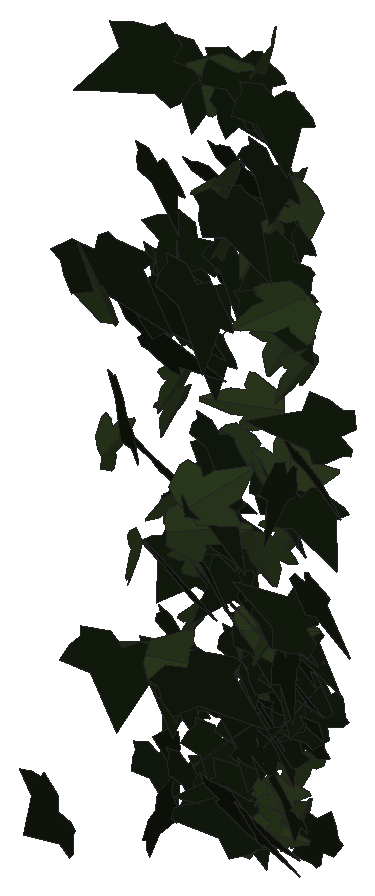
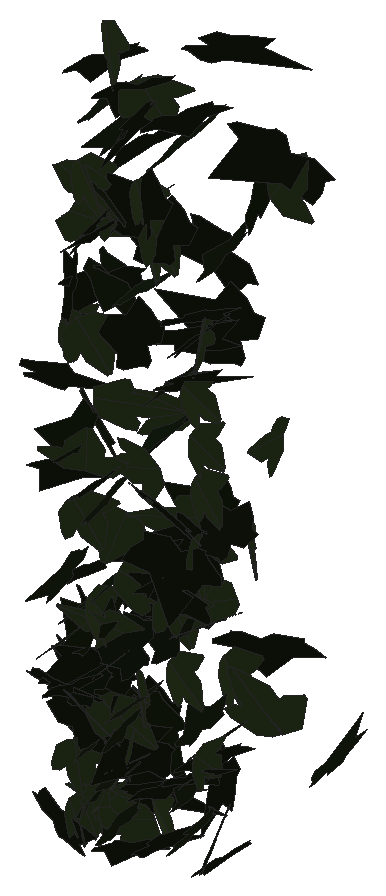
# SketchUp Ruby script. Lengths in inches.
U = 1.inch
M = Sketchup.active_model
def pt(a) = Geom::Point3d.new(a.map { |v| v * U })
def face(e, loops, mat)
  f = e.add_face(loops[0].map { |a| pt(a) })
  loops[1..].each { |l| e.add_face(l.map { |a| pt(a) }).erase! }
  f.material = f.back_material = mat if mat
  f
end
# faces: each face lists its corners as indices into pts; further lists are holes
def faces(e, pts, list, mat = nil) = list.each { |f| face(e, (f[0].is_a?(Array) ? f : [f]).map { |l| l.map { |i| pts[i] } }, mat) }
# xy, xz, yz: faces in a plane at the given z, y or x. An outline is a flat list of corners, or four numbers for a rectangle; further outlines are holes
def ring(l) = l.size == 4 ? [[l[0], l[1]], [l[2], l[1]], [l[2], l[3]], [l[0], l[3]]] : l.each_slice(2).to_a
def flat(e, list, mat, &to3) = list.each { |f| face(e, (f[0].is_a?(Array) ? f : [f]).map { |l| ring(l).map { |u, v| to3.(u, v) } }, mat) }
def xy(e, z, list, mat = nil) = flat(e, list, mat) { |x, y| [x, y, z] }
def xz(e, y, list, mat = nil) = flat(e, list, mat) { |x, z| [x, y, z] }
def yz(e, x, list, mat = nil) = flat(e, list, mat) { |y, z| [x, y, z] }
def lines(e, pts, list) = list.each { |a, b| e.add_line(pt(pts[a]), pt(pts[b])) }
# prism: a flat outline (further loops are holes) pulled along v
def prism(e, loops, v, mat = nil)
  f = face(e, loops, mat); d = Geom::Vector3d.new(v.map { |x| x * U })
  f.pushpull(f.normal.samedirection?(d) ? d.length : -d.length)
end
def box(e, o, s, mat = nil) = prism(e, [[o, [o[0] + s[0], o[1], o[2]], [o[0] + s[0], o[1] + s[1], o[2]], [o[0], o[1] + s[1], o[2]]]], [0, 0, s[2]], mat)
def at(x, y, z, deg = 0) = Geom::Transformation.translation(pt([x, y, z])) * Geom::Transformation.rotation(ORIGIN, Z_AXIS, deg.degrees)
def axes(o, x, y, z) = Geom::Transformation.new([*x, 0, *y, 0, *z, 0, *pt(o).to_a, 1])
def part(name) = M.definitions.add(name)
# library, detail: a bought-in or finely detailed component or shape, given as its bounding box
def library(name, o, s) = part(name).tap { |d| box(d.entities, o, s) }
def detail(e, o, s) = box(e.add_group.entities, o, s)
def put(e, d, t, mat = nil) = e.add_instance(d, t).tap { |i| i.material = mat if mat }
def group(e, t, mat = nil) = e.add_group.tap { |g| g.transformation = t; g.material = mat if mat }.entities
root = M.entities
M.materials.add("1026 AP 7946 SUNNY SIDE UP").color = [254, 231, 186]
M.materials.add("efeu1").color = [18, 25, 13]
M.materials.add("efeu2").color = [43, 57, 29]
c1 = part("ivyleaf_10")
p = [[0,0.5,-0.03],[-0.0625,2.02,-0.43],[-0.19,2.01,-0.46],[-0.54,1.05,-0.29],[-0.52,0.625,-0.18],[-0.83,0.76,-0.28],
  [-1.16,0.64,-0.33],[-1.15,0.33,-0.24],[-0.77,-0.39,0.02],[-0.3,-0.51,0.16],[0.04,-0.48,0.23],[-0.02,2.01,-0.4375],
  [-0.06,2.01,-0.43],[0.04,-0.49,0.23],[0.67,-0.49,0.14],[1.38,0.36,-0.2],[1.375,0.51,-0.24],[0.81,0.65,-0.19],
  [0.62,0.59,-0.15],[0.6,1.09,-0.28],[0.5,1.23,-0.31]]
faces(c1.entities,p,[[0,1,2,3,4,5,6,7,8,9,10],[11,12,0,13,14,15,16,17,18,19,20]],"efeu2")
c2 = part("ivyleaf_9")
p = [[1.54,2.16,1.25],[1.36,2.04,1.19],[-0.21,0.99,0.68],[-0.71,1.11,0.82],[-0.85,0.86,0.67],[-0.8,0.17,0.21],
  [-0.9,-0.01,0.1],[-0.67,-0.16,-0.02],[-0.08,-0.08,-0.05],[-0.03,-0.6,-0.4],[0.65,-0.88,-0.66],[0.83,-0.6,-0.49],
  [1.29,-0.42,-0.43],[1.8125,-0.07,-0.26],[1.21,0.44,0.15]]
faces(c2.entities,p,[[0,1,2,3,4,5,6,7,8,9,10,11,12,13,14]],"efeu1")
put(root,c1,axes([108.21,211.42,269.92],[-0.38508,-0.11974,0.18421],[0.25693,0.07439,0.28124],[-0.22157,0.29438,0.00598]),"1026 AP 7946 SUNNY SIDE UP")
put(root,c2,axes([108.45,212.45,268.24],[-0.09112,0.03942,0.27025],[-0.12592,-0.25836,0.02028],[0.39729,-0.07284,0.06841]),"1026 AP 7946 SUNNY SIDE UP")
put(root,c2,axes([108.26,212.3125,276.96],[0.1139,-0.28352,0.10218],[0.01275,-0.1018,-0.30159],[0.47298,0.07102,-0.01647]),"1026 AP 7946 SUNNY SIDE UP")
put(root,c1,axes([108.5,212.45,273.58],[0.01567,-0.27591,0.10372],[0.02815,-0.10155,-0.28469],[0.46182,0.01555,0.01384]),"1026 AP 7946 SUNNY SIDE UP")
put(root,c2,axes([108.35,212.22,268.26],[0.03152,-0.26953,-0.01684],[0,0.01486,-0.27835],[0.42445,0.02002,0.00125]),"1026 AP 7946 SUNNY SIDE UP")
put(root,c1,axes([108.45,212.51,269.73],[-0.0271,-0.18167,0.22393],[0.11944,-0.21378,-0.17827],[0.43042,0.04789,0.06357]),"1026 AP 7946 SUNNY SIDE UP")
put(root,c2,axes([108.48,209.94,268.49],[-0.15512,-0.1523,0.33154],[-0.07342,-0.3264,-0.17532],[0.55625,-0.08556,0.06931]),"1026 AP 7946 SUNNY SIDE UP")
put(root,c1,axes([108.59,210.81,273.55],[0.01808,0.03987,-0.32698],[0.09158,0.31227,0.04438],[0.49495,-0.05923,0.00374]),"1026 AP 7946 SUNNY SIDE UP")
put(root,c1,axes([108.64,212.47,274.91],[0.03982,-0.23204,0.18636],[0.02591,-0.18149,-0.24152],[0.4632,0.0301,-0.00251]),"1026 AP 7946 SUNNY SIDE UP")
put(root,c2,axes([108.54,212.25,269.64],[-0.10608,-0.28832,-0.00645],[0.01244,0.0029,-0.30494],[0.45324,-0.06756,0.00686]),"1026 AP 7946 SUNNY SIDE UP")
put(root,c2,axes([108.5,212.14,269.85],[0.02076,-0.27844,0.0287],[-0.00017,-0.02948,-0.28733],[0.44026,0.01312,-0.00146]),"1026 AP 7946 SUNNY SIDE UP")
put(root,c2,axes([108.36,212.08,272.72],[0.02547,-0.15199,0.26034],[0.2298,-0.21663,-0.14466],[0.40408,0.13278,0.06586]),"1026 AP 7946 SUNNY SIDE UP")
put(root,c1,axes([108.64,212.22,275.74],[0.10842,-0.25066,-0.15622],[0.06657,0.16128,-0.25628],[0.45464,0.03616,0.07478]),"1026 AP 7946 SUNNY SIDE UP")
put(root,c2,axes([108.85,212.52,275.01],[-0.31926,-0.0955,0.20724],[-0.20456,-0.17092,-0.21927],[0.28513,-0.22956,0.07473]),"1026 AP 7946 SUNNY SIDE UP")
put(root,c1,axes([108.6875,212.27,274.09],[0.00841,-0.22697,0.19007],[0.05005,-0.18427,-0.23394],[0.45848,0.02428,0.02205]),"1026 AP 7946 SUNNY SIDE UP")
put(root,c2,axes([108.74,212.47,275.97],[-0.29125,-0.2036,0.1153],[-0.04572,-0.12313,-0.27819],[0.36333,-0.1787,0.05742]),"1026 AP 7946 SUNNY SIDE UP")
put(root,c2,axes([108.72,212.46,269.38],[-0.22926,-0.20854,0.0696],[-0.01866,-0.07491,-0.26049],[0.34476,-0.14273,0.03218]),"1026 AP 7946 SUNNY SIDE UP")
put(root,c2,axes([108.56,212.39,270.1],[0.02886,-0.22884,0.17961],[0.06645,-0.17196,-0.23637],[0.44871,0.04019,0.02346]),"1026 AP 7946 SUNNY SIDE UP")
put(root,c2,axes([108.59,212.24,269.48],[0.11709,-0.26504,-0.00957],[-0.0023,0.00768,-0.28356],[0.41692,0.07448,0.00112]),"1026 AP 7946 SUNNY SIDE UP")
put(root,c2,axes([108.625,212.42,269.23],[0.11304,-0.25356,0.08159],[0.01761,-0.08057,-0.27176],[0.41801,0.07197,-0.01061]),"1026 AP 7946 SUNNY SIDE UP")
put(root,c2,axes([108.8,212.22,271.37],[-0.20416,-0.21499,0.13414],[-0.01633,-0.14316,-0.25266],[0.39588,-0.11678,0.05875]),"1026 AP 7946 SUNNY SIDE UP")
put(root,c1,axes([108.85,211.95,272.4],[-0.08755,-0.29398,-0.07375],[0.04188,0.06604,-0.30754],[0.47331,-0.06022,0.01357]),"1026 AP 7946 SUNNY SIDE UP")
put(root,c2,axes([108.67,212.25,275.67],[0.08604,-0.298,-0.03228],[-0.0153,0.02834,-0.31193],[0.47064,0.0554,-0.00424]),"1026 AP 7946 SUNNY SIDE UP")
put(root,c2,axes([109.18,211.39,279.24],[-0.46035,-0.12319,0.18772],[-0.24253,-0.10291,-0.32633],[0.24784,-0.32952,0.02935]),"1026 AP 7946 SUNNY SIDE UP")
put(root,c2,axes([108.83,210.85,270.6],[-0.32112,-0.25471,-0.11661],[0.1453,0.06862,-0.33472],[0.41251,-0.22245,0.02713]),"1026 AP 7946 SUNNY SIDE UP")
put(root,c1,axes([108.98,211.25,270.29],[0.02619,-0.33234,0.09783],[0.0047,-0.09682,-0.34337],[0.5443,0.01683,-0.00174]),"1026 AP 7946 SUNNY SIDE UP")
put(root,c2,axes([109.28,211.97,275.2],[-0.4254,-0.19819,0.01138],[-0.00316,0.02331,0.34502],[-0.31221,0.26981,-0.01901]),"1026 AP 7946 SUNNY SIDE UP")
put(root,c1,axes([109.04,212.26,270.68],[0.03283,-0.26956,0.13359],[0.01045,-0.13107,-0.27928],[0.47129,0.02168,-0.00311]),"1026 AP 7946 SUNNY SIDE UP")
put(root,c2,axes([109.02,212.26,272.37],[0.32245,0.19273,-0.10985],[-0.09658,-0.09142,-0.28949],[-0.33347,0.21284,-0.02238]),"1026 AP 7946 SUNNY SIDE UP")
put(root,c1,axes([109.0625,210.85,272.1875],[0.2021,-0.2708,-0.1119],[-0.0382,0.10667,-0.30732],[0.45629,0.12887,0.02383]),"1026 AP 7946 SUNNY SIDE UP")
put(root,c2,axes([108.9375,212.37,278.75],[-0.17368,-0.30751,0.00823],[0.00534,-0.01156,-0.3366],[0.48375,-0.11028,0.00667]),"1026 AP 7946 SUNNY SIDE UP")
put(root,c1,axes([109.14,212.23,271.58],[-0.18566,-0.24349,0.08926],[-0.02236,-0.09051,-0.27808],[0.4065,-0.11618,0.02547]),"1026 AP 7946 SUNNY SIDE UP")
put(root,c2,axes([108.92,212.11,268.35],[0.09409,-0.25828,0.0604],[0.00915,-0.06031,-0.27336],[0.41687,0.05962,-0.00763]),"1026 AP 7946 SUNNY SIDE UP")
put(root,c1,axes([109.41,209.74,276.38],[-0.41079,0.20274,-0.18884],[-0.19518,0.13968,0.3401],[0.38426,0.28769,-0.02913]),"1026 AP 7946 SUNNY SIDE UP")
put(root,c1,axes([109.26,212.43,276.96],[-0.07602,-0.27745,0.10971],[0.00885,-0.11031,-0.28983],[0.46811,-0.04297,0.0233]),"1026 AP 7946 SUNNY SIDE UP")
put(root,c2,axes([109.05,212.37,271.9],[-0.22818,-0.12076,-0.23174],[0.31956,0.10069,-0.19074],[0.24142,-0.24741,0.03345]),"1026 AP 7946 SUNNY SIDE UP")
put(root,c2,axes([108.89,211.95,272.35],[0.0601,-0.04519,-0.31088],[0.47289,0.05549,0.03104],[0.07873,-0.29882,0.05093]),"1026 AP 7946 SUNNY SIDE UP")
put(root,c2,axes([109.35,212.39,268.15],[-0.2095,-0.1547,0.18511],[-0.14566,-0.15686,-0.20978],[0.34434,-0.16047,0.02389]),"1026 AP 7946 SUNNY SIDE UP")
put(root,c2,axes([109.14,212.22,271.95],[-0.04668,-0.26512,-0.10814],[0.03026,0.10192,-0.27413],[0.44647,-0.03463,0.00728]),"1026 AP 7946 SUNNY SIDE UP")
put(root,c2,axes([109.49,212.27,273.01],[-0.47,0.07295,-0.05335],[0.06885,-0.03984,-0.31589],[-0.12311,-0.3008,0.02701]),"1026 AP 7946 SUNNY SIDE UP")
put(root,c2,axes([109.14,212.25,274.76],[0.01013,-0.28119,0.09487],[0.01244,-0.09351,-0.29025],[0.46588,0.00861,0.00569]),"1026 AP 7946 SUNNY SIDE UP")
put(root,c2,axes([108.88,211.29,275.11],[0.24269,-0.12626,0.30548],[0.33277,-0.20931,-0.20603],[0.38358,0.26147,-0.01454]),"1026 AP 7946 SUNNY SIDE UP")
put(root,c2,axes([109.06,212.26,271.18],[0.2126,-0.22558,0.15947],[0.10003,-0.14348,-0.27124],[0.41957,0.14851,-0.01614]),"1026 AP 7946 SUNNY SIDE UP")
put(root,c1,axes([109.73,212.28,271.75],[-0.15956,0.00118,0.30737],[-0.43561,-0.11735,-0.09728],[0.17414,-0.29247,0.03828]),"1026 AP 7946 SUNNY SIDE UP")
put(root,c2,axes([109.5,210.74,268.5],[0.0177,-0.00007,-0.35622],[-0.37138,0.25267,-0.0065],[0.39709,0.23632,0.0098]),"1026 AP 7946 SUNNY SIDE UP")
put(root,c2,axes([109.04,212.43,276.92],[0.17425,-0.14442,0.25797],[0.30636,-0.16197,-0.1854],[0.33729,0.22173,0.03513]),"1026 AP 7946 SUNNY SIDE UP")
put(root,c1,axes([109.56,212.26,278.84],[-0.30468,-0.20546,0.14914],[-0.02088,-0.1755,-0.27374],[0.39572,-0.16745,0.10038]),"1026 AP 7946 SUNNY SIDE UP")
put(root,c2,axes([109.26,212.06,271.52],[0.06623,-0.20026,0.20276],[0.08537,-0.19063,-0.21168],[0.43446,0.06798,0.01069]),"1026 AP 7946 SUNNY SIDE UP")
put(root,c2,axes([109.41,212.1875,268.88],[-0.1118,-0.26349,0.02848],[-0.00094,-0.03001,-0.28123],[0.41683,-0.07074,0.00701]),"1026 AP 7946 SUNNY SIDE UP")
put(root,c1,axes([109.55,212.35,277.39],[0.01457,-0.31132,0.0107],[-0.00388,-0.01224,-0.32092],[0.48987,0.00916,-0.00286]),"1026 AP 7946 SUNNY SIDE UP")
put(root,c2,axes([109.18,209.91,277.04],[-0.11236,-0.0908,-0.37005],[0.43755,0.22759,-0.11513],[0.38345,-0.2863,0.02293]),"1026 AP 7946 SUNNY SIDE UP")
put(root,c1,axes([109.65,211.87,268.35],[0.14164,-0.26064,0.03875],[0.00591,-0.04004,-0.28417],[0.41438,0.08966,-0.00919]),"1026 AP 7946 SUNNY SIDE UP")
put(root,c1,axes([109.71,212,276.66],[0.07654,-0.29666,-0.08718],[-0.0175,0.08222,-0.30921],[0.48403,0.04988,0.0026]),"1026 AP 7946 SUNNY SIDE UP")
put(root,c2,axes([109.55,212.22,278.56],[0.19127,-0.19571,-0.25033],[-0.17569,0.21491,-0.23576],[0.45661,0.16468,0.01415]),"1026 AP 7946 SUNNY SIDE UP")
put(root,c1,axes([109.6875,212.21,270.34],[0.21161,-0.22872,-0.09366],[-0.00651,0.10006,-0.2689],[0.38621,0.12701,0.04678]),"1026 AP 7946 SUNNY SIDE UP")
put(root,c2,axes([109.54,212.54,270.16],[0.00895,-0.26353,0.08883],[0.0243,-0.0873,-0.27174],[0.43605,0.01027,0.01332]),"1026 AP 7946 SUNNY SIDE UP")
put(root,c1,axes([109.4,211.4,272.37],[0.03938,-0.01328,-0.34519],[0.42802,0.19691,0.01407],[0.30774,-0.27217,0.02459]),"1026 AP 7946 SUNNY SIDE UP")
put(root,c2,axes([109.32,210.91,276.02],[0.05322,-0.068,-0.32864],[0.47655,0.12411,0.00661],[0.18797,-0.2954,0.0763]),"1026 AP 7946 SUNNY SIDE UP")
put(root,c2,axes([109.6,212.34,275.97],[-0.07769,-0.26625,0.12791],[0.03977,-0.13079,-0.27599],[0.46123,-0.03357,0.04534]),"1026 AP 7946 SUNNY SIDE UP")
put(root,c2,axes([109.37,212.47,277.19],[0.14324,-0.11433,0.28617],[0.26654,-0.2209,-0.15187],[0.39109,0.19242,-0.00131]),"1026 AP 7946 SUNNY SIDE UP")
put(root,c2,axes([109.58,212.21,269.48],[0.36551,0.14994,0.05592],[0.08399,0.0156,-0.28443],[-0.23577,0.238,-0.01463]),"1026 AP 7946 SUNNY SIDE UP")
put(root,c2,axes([109.58,212.0625,272.18],[0.00854,-0.25532,-0.13761],[0.0296,0.13218,-0.26157],[0.45107,-0.00384,0.01977]),"1026 AP 7946 SUNNY SIDE UP")
put(root,c2,axes([109.62,212.36,278.94],[-0.09019,-0.28228,-0.11128],[0.05527,0.10133,-0.29583],[0.47112,-0.06593,0.0134]),"1026 AP 7946 SUNNY SIDE UP")
put(root,c2,axes([109.42,212.47,275.35],[0.24084,-0.14711,0.22529],[0.2246,-0.16738,-0.21921],[0.34959,0.20889,-0.01438]),"1026 AP 7946 SUNNY SIDE UP")
put(root,c1,axes([110.06,212.36,269.84],[-0.25809,-0.08493,0.22107],[-0.27365,-0.1283,-0.18977],[0.23942,-0.23819,0.02141]),"1026 AP 7946 SUNNY SIDE UP")
put(root,c2,axes([109.66,211.84,273.63],[0.00195,-0.26567,0.12454],[0.03045,-0.12206,-0.27385],[0.45894,0.00923,0.01764]),"1026 AP 7946 SUNNY SIDE UP")
put(root,c1,axes([109.58,212.21,273.4],[-0.22868,0.06658,-0.26236],[0.30955,-0.16627,-0.16133],[-0.27562,-0.24198,0.03648]),"1026 AP 7946 SUNNY SIDE UP")
put(root,c2,axes([109.95,211.85,271.72],[-0.41933,0.06974,-0.11764],[0.16197,-0.05686,-0.28297],[-0.1351,-0.28463,0.02587]),"1026 AP 7946 SUNNY SIDE UP")
put(root,c2,axes([110.07,211.91,268.45],[-0.28378,-0.04454,0.19367],[-0.23391,-0.13263,-0.18002],[0.19445,-0.22454,0.06609]),"1026 AP 7946 SUNNY SIDE UP")
put(root,c2,axes([109.74,212.3,267.99],[-0.08597,-0.23886,-0.09536],[0.09497,0.07856,-0.2488],[0.39065,-0.07166,0.0395]),"1026 AP 7946 SUNNY SIDE UP")
put(root,c1,axes([109.68,212.45,269.27],[-0.01198,-0.03394,0.28348],[0.31436,-0.19168,-0.01976],[0.3025,0.19785,0.03177]),"1026 AP 7946 SUNNY SIDE UP")
put(root,c1,axes([110.18,212.16,274.11],[-0.02696,0.0521,0.30951],[-0.33256,-0.21839,0.02533],[0.34474,-0.2066,0.04864]),"1026 AP 7946 SUNNY SIDE UP")
put(root,c2,axes([109.81,212.37,269.1],[-0.09699,-0.26572,0.04503],[-0.00674,-0.04541,-0.28122],[0.42377,-0.06154,0.00583]),"1026 AP 7946 SUNNY SIDE UP")
put(root,c1,axes([109.66,210.7,270.82],[0.03202,0.08779,0.34852],[0.24598,0.3002,-0.08833],[-0.49061,0.15624,-0.02154]),"1026 AP 7946 SUNNY SIDE UP")
put(root,c2,axes([109.58,210.86,272.08],[0.16669,-0.19976,0.23086],[0.19792,-0.1875,-0.23345],[0.43002,0.16374,0.01796]),"1026 AP 7946 SUNNY SIDE UP")
put(root,c2,axes([110.14,211.49,269.47],[-0.14682,0.33268,-0.04543],[0.00405,-0.04702,-0.35609],[-0.52806,-0.09286,0.0099]),"1026 AP 7946 SUNNY SIDE UP")
put(root,c2,axes([109.66,212.26,270.82],[0.34965,-0.18247,0.06917],[0.06709,-0.05533,-0.29624],[0.29885,0.22591,-0.01443]),"1026 AP 7946 SUNNY SIDE UP")
put(root,c2,axes([109.82,212.46,269.01],[-0.02414,-0.22307,0.16609],[0.03491,-0.16321,-0.22962],[0.43254,0.00072,0.0278]),"1026 AP 7946 SUNNY SIDE UP")
put(root,c2,axes([109.79,211.98,277],[0.14011,-0.28914,-0.08488],[-0.02837,0.07893,-0.31117],[0.47118,0.09073,0.0065]),"1026 AP 7946 SUNNY SIDE UP")
put(root,c2,axes([109.76,212.42,269.72],[0.18173,-0.24131,0.08075],[0.02496,-0.08059,-0.27537],[0.39884,0.11499,-0.01956]),"1026 AP 7946 SUNNY SIDE UP")
put(root,c2,axes([109.76,212.41,278.33],[0.23751,-0.26749,-0.0068],[-0.00904,0.00259,-0.31643],[0.42058,0.15111,-0.00296]),"1026 AP 7946 SUNNY SIDE UP")
put(root,c2,axes([110.34,211.55,268.31],[-0.1146,-0.10404,-0.27909],[-0.29114,-0.19762,0.12863],[-0.35024,0.19832,-0.0156]),"1026 AP 7946 SUNNY SIDE UP")
put(root,c2,axes([110.22,212.33,277.22],[-0.39628,0.15183,-0.09006],[0.09583,-0.06922,-0.30226],[-0.259,-0.25791,0.02596]),"1026 AP 7946 SUNNY SIDE UP")
put(root,c2,axes([109.88,212.38,268.24],[0.07974,-0.22847,0.11688],[0.03851,-0.11211,-0.24176],[0.40017,0.05632,-0.00002]),"1026 AP 7946 SUNNY SIDE UP")
put(root,c2,axes([109.89,212.29,270.66],[0.10699,-0.28889,0.0015],[-0.0047,-0.00388,-0.30575],[0.45425,0.068,-0.00351]),"1026 AP 7946 SUNNY SIDE UP")
put(root,c1,axes([110.16,212.24,279.42],[0.05921,-0.28591,-0.13336],[-0.028,0.12659,-0.29634],[0.49166,0.04164,-0.00082]),"1026 AP 7946 SUNNY SIDE UP")
put(root,c2,axes([110.43,212.02,269.05],[0.07162,-0.0013,0.30492],[-0.42059,0.12807,0.04373],[-0.19932,-0.27071,0.01729]),"1026 AP 7946 SUNNY SIDE UP")
put(root,c2,axes([110.34,212.125,275.95],[-0.28119,0.24603,-0.14546],[0.10779,-0.12618,-0.31359],[-0.43395,-0.19077,0.01636]),"1026 AP 7946 SUNNY SIDE UP")
put(root,c2,axes([110.11,212,271.27],[-0.11348,-0.02272,0.3238],[-0.04618,-0.32069,-0.03269],[0.49356,-0.03523,0.07139]),"1026 AP 7946 SUNNY SIDE UP")
put(root,c1,axes([110.19,212.2,268.3],[-0.02453,-0.06083,0.27098],[0.06767,-0.26102,-0.061],[0.41963,0.03854,0.02568]),"1026 AP 7946 SUNNY SIDE UP")
put(root,c2,axes([110.03,211.14,273.33],[0.14676,-0.33918,-0.07772],[-0.04713,0.06796,-0.36185],[0.54367,0.09745,-0.01039]),"1026 AP 7946 SUNNY SIDE UP")
put(root,c1,axes([110.25,211.92,272.26],[-0.46477,0.02747,-0.04736],[0.06762,-0.03335,-0.30456],[-0.05053,-0.29729,0.02801]),"1026 AP 7946 SUNNY SIDE UP")
put(root,c1,axes([110.3,212.02,276.82],[-0.09322,-0.24438,0.20753],[0.04351,-0.20953,-0.25296],[0.49748,-0.02747,0.06101]),"1026 AP 7946 SUNNY SIDE UP")
put(root,c2,axes([110.09,212.32,272.85],[0.21094,-0.26191,-0.06165],[-0.06049,0.0458,-0.30258],[0.41757,0.13894,-0.01269]),"1026 AP 7946 SUNNY SIDE UP")
put(root,c2,axes([110.07,210.72,270.8],[0.0275,-0.13045,-0.33785],[0.08202,0.32495,-0.12869],[0.54777,-0.04211,0.03623]),"1026 AP 7946 SUNNY SIDE UP")
put(root,c1,axes([110.39,212.44,275.18],[-0.19417,-0.26452,0.13869],[-0.02338,-0.14171,-0.29842],[0.4672,-0.11703,0.0427]),"1026 AP 7946 SUNNY SIDE UP")
put(root,c2,axes([110.2,212.49,276.6875],[-0.03919,-0.29788,0.05005],[0.0027,-0.05059,-0.30818],[0.47501,-0.02429,0.00588]),"1026 AP 7946 SUNNY SIDE UP")
put(root,c1,axes([110.39,212.43,277.45],[-0.02874,-0.30149,0.05769],[-0.00465,-0.05764,-0.3115],[0.48265,-0.01851,0.00044]),"1026 AP 7946 SUNNY SIDE UP")
put(root,c2,axes([110.16,212.1875,276.9],[0.18838,-0.2835,-0.13585],[-0.0927,0.11645,-0.31627],[0.48175,0.13327,-0.00774]),"1026 AP 7946 SUNNY SIDE UP")
put(root,c1,axes([110.04,211.82,268.01],[-0.06906,-0.05746,-0.31447],[0.45693,0.10036,-0.06201],[0.17107,-0.29127,0.03869]),"1026 AP 7946 SUNNY SIDE UP")
put(root,c2,axes([110.23,212.31,273.05],[0.05695,-0.2873,-0.02183],[-0.00957,0.01894,-0.29818],[0.45269,0.03654,-0.00356]),"1026 AP 7946 SUNNY SIDE UP")
put(root,c1,axes([110.02,212.09,270.8],[0.15649,-0.04857,-0.30446],[0.46961,0.03523,0.09795],[0.0289,-0.30958,0.05703]),"1026 AP 7946 SUNNY SIDE UP")
put(root,c1,axes([110.1875,212.17,268.43],[0.32051,0.13483,0.13631],[0.1961,0.04867,-0.25018],[-0.22198,0.23767,-0.0242]),"1026 AP 7946 SUNNY SIDE UP")
put(root,c1,axes([110.15,210.76,273.34],[0.29636,0.08956,-0.29737],[0.33224,0.205,0.2085],[0.34086,-0.27769,0.05533]),"1026 AP 7946 SUNNY SIDE UP")
put(root,c2,axes([110.68,212.23,269.68],[-0.27244,0.18609,0.08879],[-0.10962,0.05119,-0.26117],[-0.30253,-0.18614,0.01468]),"1026 AP 7946 SUNNY SIDE UP")
put(root,c1,axes([110.46,212.08,271.05],[0.02004,-0.27321,0.14388],[0.00095,-0.14131,-0.28254],[0.48359,0.0116,-0.00541]),"1026 AP 7946 SUNNY SIDE UP")
put(root,c2,axes([110.24,212.33,269.35],[0.0816,-0.25913,0.0735],[0.00166,-0.07396,-0.27236],[0.42324,0.05025,-0.0131]),"1026 AP 7946 SUNNY SIDE UP")
put(root,c1,axes([110.43,212.1,268.2],[-0.16381,0.16114,0.19891],[0.06631,-0.19387,0.18989],[0.38872,0.10097,0.05143]),"1026 AP 7946 SUNNY SIDE UP")
put(root,c2,axes([110.23,211.3125,277.54],[0.09546,-0.30985,-0.1413],[-0.00655,0.13686,-0.32379],[0.53165,0.05732,0.02138]),"1026 AP 7946 SUNNY SIDE UP")
put(root,c1,axes([110.65,212.32,277.29],[0.32631,-0.10777,-0.21612],[-0.31007,0.07252,-0.23961],[0.20188,0.28559,-0.0187]),"1026 AP 7946 SUNNY SIDE UP")
put(root,c2,axes([110.32,212.09,275.86],[-0.00934,-0.24366,-0.21528],[0.02582,0.20712,-0.24973],[0.50266,-0.01516,0.00882]),"1026 AP 7946 SUNNY SIDE UP")
put(root,c1,axes([110.4375,212.31,268.1875],[0.01029,-0.2234,0.14069],[0.12436,-0.12979,-0.22134],[0.39357,0.04685,0.06626]),"1026 AP 7946 SUNNY SIDE UP")
put(root,c1,axes([110.59,212.29,272.5],[-0.1573,-0.25475,0.1206],[-0.01451,-0.12276,-0.28058],[0.44157,-0.09479,0.03374]),"1026 AP 7946 SUNNY SIDE UP")
put(root,c1,axes([110.49,212.28,273.17],[0.45867,0.13134,-0.00243],[-0.01398,0.02729,0.32841],[0.2061,-0.29044,0.0277]),"1026 AP 7946 SUNNY SIDE UP")
put(root,c2,axes([110.36,209.01,275.4375],[0.00285,-0.11456,0.38224],[-0.02153,-0.37148,-0.12005],[0.61119,-0.01255,-0.00601]),"1026 AP 7946 SUNNY SIDE UP")
put(root,c2,axes([110.75,212.2,269.3],[0.13598,-0.10271,0.29659],[-0.23937,0.24568,0.13856],[-0.41779,-0.17419,0.01715]),"1026 AP 7946 SUNNY SIDE UP")
put(root,c2,axes([110.3,212.25,270.36],[-0.05339,-0.1265,-0.26751],[0.27829,0.19664,-0.12172],[0.35766,-0.17188,0.05477]),"1026 AP 7946 SUNNY SIDE UP")
put(root,c1,axes([110.64,212.29,269.01],[-0.2225,-0.22586,0.00715],[0.01079,-0.01399,-0.27432],[0.35522,-0.14105,0.01281]),"1026 AP 7946 SUNNY SIDE UP")
put(root,c2,axes([110.54,212.47,270.07],[-0.15947,-0.25005,0.02071],[0.00265,-0.0239,-0.27792],[0.39463,-0.10089,0.01024]),"1026 AP 7946 SUNNY SIDE UP")
put(root,c2,axes([110.42,211.88,271.3125],[0.25405,-0.18457,-0.15179],[-0.08992,0.14136,-0.24796],[0.35924,0.16591,0.04528]),"1026 AP 7946 SUNNY SIDE UP")
put(root,c2,axes([110.4375,212.29,268.36],[0.04228,-0.19665,0.20767],[0.02097,-0.2025,-0.2054],[0.44357,0.02832,-0.01009]),"1026 AP 7946 SUNNY SIDE UP")
put(root,c2,axes([110.33,212.37,270.0625],[0.12074,-0.14432,0.22919],[0.15759,-0.19956,-0.16955],[0.38722,0.12622,-0.00246]),"1026 AP 7946 SUNNY SIDE UP")
put(root,c1,axes([110.61,212.37,268.21],[0.0116,-0.25213,0.07442],[0.05398,-0.07215,-0.25832],[0.40949,0.01665,0.03194]),"1026 AP 7946 SUNNY SIDE UP")
put(root,c2,axes([110.49,211.93,278.87],[-0.07405,-0.3054,-0.05312],[0.02983,0.04746,-0.31785],[0.48565,-0.04948,0.01142]),"1026 AP 7946 SUNNY SIDE UP")
put(root,c2,axes([110.43,212.25,270.71],[0.06547,-0.21233,0.21891],[0.156,-0.19403,-0.21965],[0.44725,0.09876,0.04457]),"1026 AP 7946 SUNNY SIDE UP")
put(root,c2,axes([110.76,211.93,276.59],[-0.29172,-0.16255,0.18362],[-0.07662,-0.19604,-0.23637],[0.37258,-0.16759,0.09516]),"1026 AP 7946 SUNNY SIDE UP")
put(root,c2,axes([110.52,212.34,270.86],[0.19168,-0.2365,-0.10428],[-0.03457,0.10054,-0.27232],[0.4022,0.12136,0.02629]),"1026 AP 7946 SUNNY SIDE UP")
put(root,c2,axes([110.61,211.8,269.57],[0.0362,0.28742,0.08722],[-0.04196,-0.08097,0.2959],[0.46854,-0.02946,0.01976]),"1026 AP 7946 SUNNY SIDE UP")
put(root,c2,axes([110.49,212.58,275.78],[0.14154,-0.13552,-0.28489],[0.4058,-0.12262,0.14815],[-0.26223,-0.2629,0.07548]),"1026 AP 7946 SUNNY SIDE UP")
put(root,c2,axes([110.5625,210.24,276.86],[0.01276,-0.37332,0.14739],[-0.00236,-0.14525,-0.3855],[0.62983,0.00702,-0.00443]),"1026 AP 7946 SUNNY SIDE UP")
put(root,c1,axes([110.8,212.19,274.97],[-0.01586,-0.2067,0.22175],[0.0245,-0.21661,-0.21365],[0.46994,0.00431,0.01862]),"1026 AP 7946 SUNNY SIDE UP")
put(root,c2,axes([110.63,211.72,278.03],[-0.04419,-0.26641,0.1575],[0.01718,-0.15581,-0.27582],[0.48387,-0.0188,0.02418]),"1026 AP 7946 SUNNY SIDE UP")
put(root,c2,axes([111.03,212.22,267.83],[-0.03116,0.06775,0.28277],[-0.21993,0.23633,-0.06922],[-0.38566,-0.14025,0.01663]),"1026 AP 7946 SUNNY SIDE UP")
put(root,c2,axes([110.98,211.92,271.24],[-0.10699,-0.29303,-0.04412],[-0.02579,-0.03843,0.30959],[-0.46456,0.06962,-0.00703]),"1026 AP 7946 SUNNY SIDE UP")
put(root,c2,axes([111.125,212.1875,269.73],[-0.38614,-0.03772,-0.13944],[-0.21614,0.01009,0.25449],[-0.04421,0.28012,-0.02628]),"1026 AP 7946 SUNNY SIDE UP")
put(root,c2,axes([110.4,211.01,268.83],[0.28939,-0.17563,0.24474],[0.26813,-0.16686,-0.26304],[0.38091,0.25089,-0.00078]),"1026 AP 7946 SUNNY SIDE UP")
put(root,c2,axes([110.68,211.92,270.73],[-0.13237,-0.03325,-0.29654],[0.44123,-0.08333,-0.07516],[-0.11243,-0.28791,0.05415]),"1026 AP 7946 SUNNY SIDE UP")
put(root,c2,axes([110.83,211.72,273.5],[-0.29112,0.01007,-0.26738],[0.37314,-0.1232,-0.17999],[-0.16629,-0.2941,0.06422]),"1026 AP 7946 SUNNY SIDE UP")
put(root,c2,axes([110.63,212.26,273.52],[0.21822,-0.23049,0.11331],[0.08295,-0.09813,-0.2777],[0.39383,0.14839,-0.00429]),"1026 AP 7946 SUNNY SIDE UP")
put(root,c1,axes([111.1,211.57,276.24],[0.24557,0.09563,-0.30341],[-0.34622,-0.1985,-0.18749],[-0.34351,0.26842,-0.02793]),"1026 AP 7946 SUNNY SIDE UP")
put(root,c2,axes([110.72,212.33,271.56],[0.25713,-0.24968,-0.04622],[-0.04494,0.03321,-0.30722],[0.39595,0.16591,-0.00485]),"1026 AP 7946 SUNNY SIDE UP")
put(root,c2,axes([111.35,212.14,274.12],[-0.32223,0.04248,0.21478],[-0.33418,-0.04308,-0.20666],[0.00245,-0.28897,0.06062]),"1026 AP 7946 SUNNY SIDE UP")
put(root,c2,axes([110.65,211.02,268.72],[0.2834,-0.18119,0.18248],[0.16736,-0.14451,-0.26318],[0.36282,0.20819,-0.02114]),"1026 AP 7946 SUNNY SIDE UP")
put(root,c2,axes([110.83,212.1,272.98],[-0.08479,-0.23789,-0.1647],[0.14028,0.13926,-0.24574],[0.42706,-0.09298,0.04802]),"1026 AP 7946 SUNNY SIDE UP")
